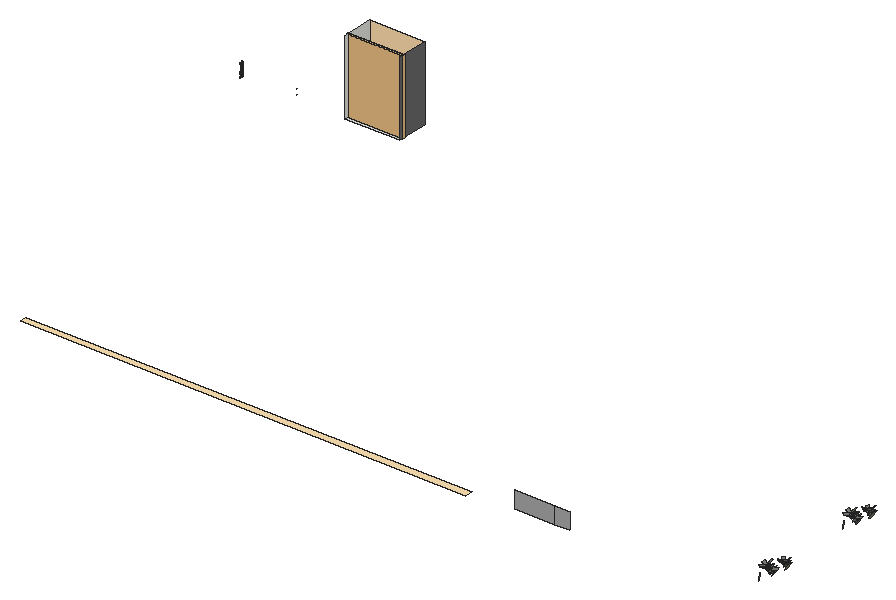
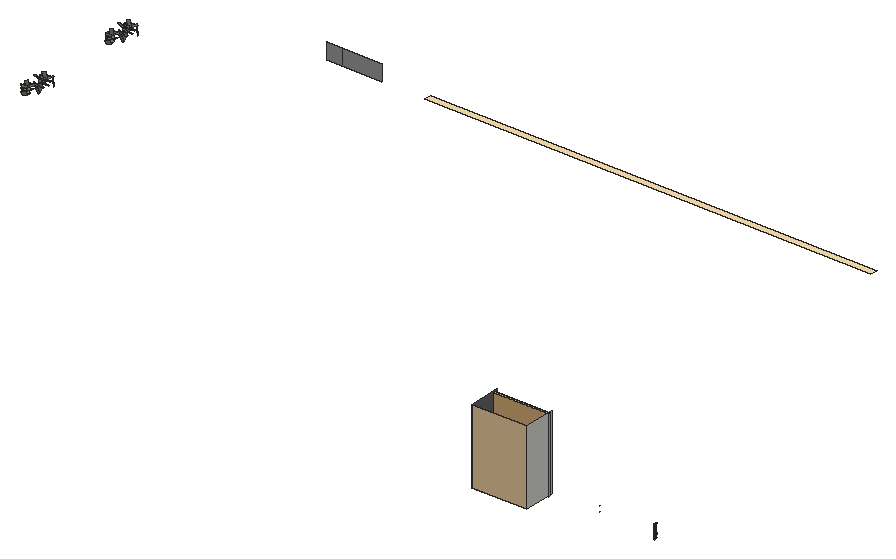
# SketchUp Ruby script. Lengths in inches.
U = 1.inch
M = Sketchup.active_model
def pt(a) = Geom::Point3d.new(a.map { |v| v * U })
def face(e, loops, mat)
  f = e.add_face(loops[0].map { |a| pt(a) })
  loops[1..].each { |l| e.add_face(l.map { |a| pt(a) }).erase! }
  f.material = f.back_material = mat if mat
  f
end
# faces: each face lists its corners as indices into pts; further lists are holes
def faces(e, pts, list, mat = nil) = list.each { |f| face(e, (f[0].is_a?(Array) ? f : [f]).map { |l| l.map { |i| pts[i] } }, mat) }
# xy, xz, yz: faces in a plane at the given z, y or x. An outline is a flat list of corners, or four numbers for a rectangle; further outlines are holes
def ring(l) = l.size == 4 ? [[l[0], l[1]], [l[2], l[1]], [l[2], l[3]], [l[0], l[3]]] : l.each_slice(2).to_a
def flat(e, list, mat, &to3) = list.each { |f| face(e, (f[0].is_a?(Array) ? f : [f]).map { |l| ring(l).map { |u, v| to3.(u, v) } }, mat) }
def xy(e, z, list, mat = nil) = flat(e, list, mat) { |x, y| [x, y, z] }
def xz(e, y, list, mat = nil) = flat(e, list, mat) { |x, z| [x, y, z] }
def yz(e, x, list, mat = nil) = flat(e, list, mat) { |y, z| [x, y, z] }
def lines(e, pts, list) = list.each { |a, b| e.add_line(pt(pts[a]), pt(pts[b])) }
# prism: a flat outline (further loops are holes) pulled along v
def prism(e, loops, v, mat = nil)
  f = face(e, loops, mat); d = Geom::Vector3d.new(v.map { |x| x * U })
  f.pushpull(f.normal.samedirection?(d) ? d.length : -d.length)
end
def box(e, o, s, mat = nil) = prism(e, [[o, [o[0] + s[0], o[1], o[2]], [o[0] + s[0], o[1] + s[1], o[2]], [o[0], o[1] + s[1], o[2]]]], [0, 0, s[2]], mat)
def at(x, y, z, deg = 0) = Geom::Transformation.translation(pt([x, y, z])) * Geom::Transformation.rotation(ORIGIN, Z_AXIS, deg.degrees)
def axes(o, x, y, z) = Geom::Transformation.new([*x, 0, *y, 0, *z, 0, *pt(o).to_a, 1])
def part(name) = M.definitions.add(name)
# library, detail: a bought-in or finely detailed component or shape, given as its bounding box
def library(name, o, s) = part(name).tap { |d| box(d.entities, o, s) }
def detail(e, o, s) = box(e.add_group.entities, o, s)
def put(e, d, t, mat = nil) = e.add_instance(d, t).tap { |i| i.material = mat if mat }
def group(e, t, mat = nil) = e.add_group.tap { |g| g.transformation = t; g.material = mat if mat }.entities
root = M.entities
M.materials.add("Material \#1").color = [140, 140, 140]
M.materials.add("[0032_Moccasin]").color = [255, 228, 181]
M.materials.add("[0033_NavajoWhite]").color = [255, 222, 173]
M.materials.add("[0132_LightGray]").color = [169, 169, 169]
M.materials.add("[0134_DimGray]").color = [105, 105, 105]
M.materials.add("viburnumblaasdfas0df1w06d").color = [98, 102, 84]
M.materials.add("viburnumbladsadfasdfad0w122").color = [125, 129, 119]
c1 = library("Glazed double door",[0,0,0],[5.31,78.43,99.16])
c2 = part("Component\#315")
p = [[0.25,0,0],[2.05,0.01,0.35],[1.81,4.2,1.66],[0,4.19,1.3125]]
faces(c2.entities,p,[[0,1,2,3]],"viburnumbladsadfasdfad0w122")
c3 = part("viburnumblad2")
put(c3.entities,c2,axes([-19.23,-4.49,-32.18],[83.35428,0,0],[0,79.38502,0],[0,0,83.35428]))
c4 = part("Component\#314")
p = [[0.14,0,0],[2.58,0.05,0.25],[2.44,5.11,2.64],[0,5.05,2.39]]
faces(c4.entities,p,[[0,1,2,3]],"viburnumblaasdfas0df1w06d")
c5 = part("viburnumblad1\#2")
put(c5.entities,c4,axes([-37.25,6.23,19.31],[75.98784,0,0],[0,65.50676,0],[0,0,75.98784]))
xy(root,40.75,[[1668.9174,528.0625,1708.7299,550.875]])
xy(root,42.5175,[[1632.1242,529.8706,1632.0426,529.8912,1632.0551,529.9063],[1632.1242,529.8706,1632.0551,529.9063,1632.1285,529.8877],[1632.1242,529.8706,1632.1285,529.8877,1632.211,529.8706],[1632.211,529.8706,1632.1285,529.8877,1632.2067,529.8877],[1632.211,529.8706,1632.2067,529.8877,1632.2926,529.8912],
  [1632.2067,529.8877,1632.2801,529.9063,1632.2926,529.8912],[1632.0426,529.8912,1631.9761,529.93,1631.9953,529.9411],[1632.0426,529.8912,1631.9953,529.9411,1632.0551,529.9063],[1632.2926,529.8912,1632.2801,529.9063,1632.3591,529.93],[1632.2801,529.9063,1632.34,529.9411,1632.3591,529.93],
  [1631.9761,529.93,1631.9327,529.9822,1631.9562,529.9881],[1631.9761,529.93,1631.9562,529.9881,1631.9953,529.9411],[1632.3591,529.93,1632.34,529.9411,1632.4025,529.9822],[1632.34,529.9411,1632.379,529.9881,1632.4025,529.9822],[1631.9327,529.9822,1631.9176,530.0416,1631.9426,530.0416],
  [1631.9327,529.9822,1631.9426,530.0416,1631.9562,529.9881],[1632.4025,529.9822,1632.379,529.9881,1632.4176,530.0416],[1632.379,529.9881,1632.3926,530.0416,1632.4176,530.0416],[1631.9176,530.0416,1631.9327,530.1009,1631.9562,530.095],[1631.9176,530.0416,1631.9562,530.095,1631.9426,530.0416],
  [1632.3926,530.0416,1632.379,530.095,1632.4025,530.1009],[1632.3926,530.0416,1632.4025,530.1009,1632.4176,530.0416],[1631.9562,530.095,1631.9327,530.1009,1631.9953,530.142],[1632.379,530.095,1632.34,530.142,1632.3591,530.1532],[1632.379,530.095,1632.3591,530.1532,1632.4025,530.1009],
  [1631.9327,530.1009,1631.9761,530.1532,1631.9953,530.142],[1631.9953,530.142,1631.9761,530.1532,1632.0551,530.1769],[1632.34,530.142,1632.2801,530.1769,1632.2926,530.1919],[1632.34,530.142,1632.2926,530.1919,1632.3591,530.1532],[1631.9761,530.1532,1632.0426,530.1919,1632.0551,530.1769],
  [1632.0551,530.1769,1632.0426,530.1919,1632.1285,530.1954],[1632.2801,530.1769,1632.2067,530.1954,1632.211,530.2125],[1632.2801,530.1769,1632.211,530.2125,1632.2926,530.1919],[1632.0426,530.1919,1632.1242,530.2125,1632.1285,530.1954],[1632.1285,530.1954,1632.1242,530.2125,1632.2067,530.1954],
  [1632.2067,530.1954,1632.1242,530.2125,1632.211,530.2125]],"Material \#1")
xy(root,42.5353,[[1632.1242,529.8706,1632.1285,529.8877,1632.0426,529.8912],[1632.1242,529.8706,1632.2067,529.8877,1632.1285,529.8877],[1632.1242,529.8706,1632.211,529.8706,1632.2067,529.8877],[1632.211,529.8706,1632.2801,529.9063,1632.2067,529.8877],[1632.211,529.8706,1632.2926,529.8912,1632.2801,529.9063],
  [1632.1285,529.8877,1632.0551,529.9063,1632.0426,529.8912],[1632.0426,529.8912,1632.0551,529.9063,1631.9761,529.93],[1632.2926,529.8912,1632.34,529.9411,1632.2801,529.9063],[1632.2926,529.8912,1632.3591,529.93,1632.34,529.9411],[1632.0551,529.9063,1631.9953,529.9411,1631.9761,529.93],
  [1631.9761,529.93,1631.9953,529.9411,1631.9327,529.9822],[1632.3591,529.93,1632.379,529.9881,1632.34,529.9411],[1632.3591,529.93,1632.4025,529.9822,1632.379,529.9881],[1631.9953,529.9411,1631.9562,529.9881,1631.9327,529.9822],[1631.9327,529.9822,1631.9562,529.9881,1631.9176,530.0416],
  [1632.4025,529.9822,1632.3926,530.0416,1632.379,529.9881],[1632.4025,529.9822,1632.4176,530.0416,1632.3926,530.0416],[1631.9562,529.9881,1631.9426,530.0416,1631.9176,530.0416],[1631.9176,530.0416,1631.9426,530.0416,1631.9327,530.1009],[1631.9426,530.0416,1631.9562,530.095,1631.9327,530.1009],
  [1632.3926,530.0416,1632.4176,530.0416,1632.379,530.095],[1632.4176,530.0416,1632.4025,530.1009,1632.379,530.095],[1631.9562,530.095,1631.9761,530.1532,1631.9327,530.1009],[1631.9562,530.095,1631.9953,530.142,1631.9761,530.1532],[1632.379,530.095,1632.4025,530.1009,1632.34,530.142],
  [1632.4025,530.1009,1632.3591,530.1532,1632.34,530.142],[1631.9953,530.142,1632.0426,530.1919,1631.9761,530.1532],[1631.9953,530.142,1632.0551,530.1769,1632.0426,530.1919],[1632.34,530.142,1632.3591,530.1532,1632.2801,530.1769],[1632.3591,530.1532,1632.2926,530.1919,1632.2801,530.1769],
  [1632.0551,530.1769,1632.1242,530.2125,1632.0426,530.1919],[1632.0551,530.1769,1632.1285,530.1954,1632.1242,530.2125],[1632.2801,530.1769,1632.2926,530.1919,1632.2067,530.1954],[1632.2926,530.1919,1632.211,530.2125,1632.2067,530.1954],[1632.1285,530.1954,1632.211,530.2125,1632.1242,530.2125],
  [1632.1285,530.1954,1632.2067,530.1954,1632.211,530.2125]],"Material \#1")
xy(root,46.5278,[[1632.1242,529.8706,1632.0426,529.8912,1632.1286,529.8877],[1632.1242,529.8706,1632.1286,529.8877,1632.2067,529.8877],[1632.1242,529.8706,1632.2067,529.8877,1632.211,529.8706],[1632.211,529.8706,1632.2067,529.8877,1632.2801,529.9063],[1632.211,529.8706,1632.2801,529.9063,1632.2926,529.8912],
  [1632.1286,529.8877,1632.0426,529.8912,1632.0551,529.9063],[1632.0426,529.8912,1631.9761,529.93,1632.0551,529.9063],[1632.2926,529.8912,1632.2801,529.9063,1632.34,529.9411],[1632.2926,529.8912,1632.34,529.9411,1632.3591,529.93],[1632.0551,529.9063,1631.9761,529.93,1631.9953,529.9411],
  [1631.9761,529.93,1631.9327,529.9822,1631.9953,529.9411],[1632.3591,529.93,1632.34,529.9411,1632.379,529.9881],[1632.3591,529.93,1632.379,529.9881,1632.4025,529.9822],[1631.9953,529.9411,1631.9327,529.9822,1631.9562,529.9881],[1631.9327,529.9822,1631.9176,530.0416,1631.9562,529.9881],
  [1632.4025,529.9822,1632.379,529.9881,1632.3926,530.0416],[1632.4025,529.9822,1632.3926,530.0416,1632.4176,530.0416],[1631.9562,529.9881,1631.9176,530.0416,1631.9426,530.0416],[1631.9176,530.0416,1631.9327,530.1009,1631.9426,530.0416],[1631.9426,530.0416,1631.9327,530.1009,1631.9562,530.095],
  [1632.3926,530.0416,1632.379,530.095,1632.4176,530.0416],[1632.4176,530.0416,1632.379,530.095,1632.4025,530.1009],[1631.9562,530.095,1631.9327,530.1009,1631.9761,530.1532],[1631.9562,530.095,1631.9761,530.1532,1631.9953,530.142],[1632.379,530.095,1632.34,530.142,1632.4025,530.1009],
  [1632.4025,530.1009,1632.34,530.142,1632.3591,530.1532],[1631.9953,530.142,1631.9761,530.1532,1632.0426,530.1919],[1631.9953,530.142,1632.0426,530.1919,1632.0551,530.1769],[1632.34,530.142,1632.2801,530.1769,1632.3591,530.1532],[1632.3591,530.1532,1632.2801,530.1769,1632.2926,530.1919],
  [1632.0551,530.1769,1632.0426,530.1919,1632.1242,530.2125],[1632.0551,530.1769,1632.1242,530.2125,1632.1286,530.1954],[1632.2801,530.1769,1632.2067,530.1954,1632.2926,530.1919],[1632.2926,530.1919,1632.2067,530.1954,1632.211,530.2125],[1632.1286,530.1954,1632.1242,530.2125,1632.211,530.2125],
  [1632.1286,530.1954,1632.211,530.2125,1632.2067,530.1954]],"Material \#1")
xy(root,46.5456,[[1632.1242,529.8706,1632.0551,529.9063,1632.0426,529.8912],[1632.1242,529.8706,1632.1286,529.8877,1632.0551,529.9063],[1632.1242,529.8706,1632.211,529.8706,1632.1286,529.8877],[1632.211,529.8706,1632.2067,529.8877,1632.1286,529.8877],[1632.211,529.8706,1632.2926,529.8912,1632.2067,529.8877],
  [1632.2067,529.8877,1632.2926,529.8912,1632.2801,529.9063],[1632.0426,529.8912,1631.9953,529.9411,1631.9761,529.93],[1632.0426,529.8912,1632.0551,529.9063,1631.9953,529.9411],[1632.2926,529.8912,1632.3591,529.93,1632.2801,529.9063],[1632.2801,529.9063,1632.3591,529.93,1632.34,529.9411],
  [1631.9761,529.93,1631.9562,529.9881,1631.9327,529.9822],[1631.9761,529.93,1631.9953,529.9411,1631.9562,529.9881],[1632.3591,529.93,1632.4025,529.9822,1632.34,529.9411],[1632.34,529.9411,1632.4025,529.9822,1632.379,529.9881],[1631.9327,529.9822,1631.9426,530.0416,1631.9176,530.0416],
  [1631.9327,529.9822,1631.9562,529.9881,1631.9426,530.0416],[1632.4025,529.9822,1632.4176,530.0416,1632.379,529.9881],[1632.379,529.9881,1632.4176,530.0416,1632.3926,530.0416],[1631.9176,530.0416,1631.9426,530.0416,1631.9562,530.095],[1631.9176,530.0416,1631.9562,530.095,1631.9327,530.1009],
  [1632.3926,530.0416,1632.4025,530.1009,1632.379,530.095],[1632.3926,530.0416,1632.4176,530.0416,1632.4025,530.1009],[1631.9562,530.095,1631.9953,530.142,1631.9327,530.1009],[1632.379,530.095,1632.3591,530.1532,1632.34,530.142],[1632.379,530.095,1632.4025,530.1009,1632.3591,530.1532],
  [1631.9327,530.1009,1631.9953,530.142,1631.9761,530.1532],[1631.9953,530.142,1632.0551,530.1769,1631.9761,530.1532],[1632.34,530.142,1632.2926,530.1919,1632.2801,530.1769],[1632.34,530.142,1632.3591,530.1532,1632.2926,530.1919],[1631.9761,530.1532,1632.0551,530.1769,1632.0426,530.1919],
  [1632.0551,530.1769,1632.1286,530.1954,1632.0426,530.1919],[1632.2801,530.1769,1632.211,530.2125,1632.2067,530.1954],[1632.2801,530.1769,1632.2926,530.1919,1632.211,530.2125],[1632.0426,530.1919,1632.1286,530.1954,1632.1242,530.2125],[1632.1286,530.1954,1632.2067,530.1954,1632.1242,530.2125],
  [1632.2067,530.1954,1632.211,530.2125,1632.1242,530.2125]],"Material \#1")
xy(root,47.6814,[[1678.9389,218.9375,2004.7084,223.9375]],"[0032_Moccasin]")
xz(root,223.9375,[[2036.3125,48,2065.6875,60]],"[0132_LightGray]")
xz(root,529.3124,[[1591.1102,42.1281,1591.052,42.4891,1591.1077,42.5206],[1591.1102,42.1281,1591.1077,42.5206,1591.1102,42.4516],[1591.1102,42.4516,1591.1077,42.5206,1591.1121,42.4659],[1591.1102,42.4516,1591.1121,42.4659,1591.1107,42.4591],[1591.1121,42.4659,1591.1077,42.5206,1591.1542,42.562],
  [1591.1121,42.4659,1591.1179,42.478,1591.1145,42.4721],[1591.1121,42.4659,1591.1542,42.562,1591.1179,42.478],[1591.1179,42.478,1591.1542,42.562,1591.1896,42.6116],[1591.1179,42.478,1591.1896,42.6116,1591.2571,42.6891],[1591.1179,42.478,1591.2571,42.6891,1591.1221,42.4835],
  [1591.1221,42.4835,1591.2571,42.6891,1591.1273,42.4887],[1591.1273,42.4887,1591.1913,42.549,1591.1333,42.4937],[1591.1273,42.4887,1591.2571,42.6891,1591.1913,42.549],[1591.1333,42.4937,1591.1913,42.549,1591.164,42.52],[1591.1913,42.549,1591.2339,42.6147,1591.2148,42.5807],
  [1591.1913,42.549,1591.2571,42.6891,1591.2339,42.6147],[1591.1896,42.6116,1591.2122,42.6678,1591.2571,42.6891],[1591.2339,42.6147,1591.2571,42.6891,1591.2482,42.6509],[1591.2122,42.6678,1591.2202,42.729,1591.2571,42.6891],[1591.2571,42.6891,1591.1854,42.9182,1591.2512,42.7983],
  [1591.2571,42.6891,1591.1896,42.8463,1591.1854,42.9182],[1591.2571,42.6891,1591.2122,42.7902,1591.1896,42.8463],[1591.2571,42.6891,1591.2202,42.729,1591.2122,42.7902],[1591.2571,42.6891,1591.2512,42.7983,1591.2602,42.7289],[1591.2512,42.7983,1591.1854,42.9182,1591.2256,42.862],
  [1591.1896,42.8463,1591.1542,42.8959,1591.1854,42.9182],[1591.1542,42.8959,1591.1077,42.9373,1591.1854,42.9182],[1591.1854,42.9182,1590.9202,43.0316,1591.0696,43.0008],[1591.1854,42.9182,1591.052,42.9688,1590.9202,43.0316],[1591.1854,42.9182,1591.1077,42.9373,1591.052,42.9688],
  [1591.1854,42.9182,1591.0696,43.0008,1591.1327,42.9651]],"Material \#1")
xz(root,529.3472,[[1591.1073,39.5491,1591.0976,39.5594,1591.1308,39.5889],[1591.1073,39.5491,1591.1308,39.5889,1591.1423,39.5802],[1591.5889,39.557,1591.5774,39.5657,1591.6622,39.6725],[1591.5889,39.557,1591.6622,39.6725,1591.6752,39.6657],[1591.1423,39.5802,1591.1308,39.5889,1591.1579,39.6231],
  [1591.1423,39.5802,1591.1579,39.6231,1591.1709,39.6163],[1591.1709,39.6163,1591.1579,39.6231,1591.1784,39.6614],[1591.1709,39.6163,1591.1784,39.6614,1591.1925,39.6567],[1591.1925,39.6567,1591.1784,39.6614,1591.1912,39.703],[1591.1925,39.6567,1591.1912,39.703,1591.2061,39.7006],
  [1591.6752,39.6657,1591.6622,39.6725,1591.7258,39.7916],[1591.6752,39.6657,1591.7258,39.7916,1591.7399,39.7869],[1591.2061,39.7006,1591.1912,39.703,1591.1957,39.7468],[1591.2061,39.7006,1591.1957,39.7468,1591.2107,39.7468],[1591.1957,39.7468,1591.1912,39.7907,1591.2107,39.7468],
  [1591.2107,39.7468,1591.1912,39.7907,1591.2061,39.7931],[1591.7399,39.7869,1591.7258,39.7916,1591.7657,39.9208],[1591.7399,39.7869,1591.7657,39.9208,1591.7805,39.9184],[1591.1912,39.7907,1591.1784,39.8323,1591.2061,39.7931],[1591.2061,39.7931,1591.1784,39.8323,1591.1925,39.837],
  [1591.1784,39.8323,1591.1579,39.8706,1591.1925,39.837],[1591.1925,39.837,1591.1579,39.8706,1591.1709,39.8774],[1591.1579,39.8706,1591.1308,39.9048,1591.1709,39.8774],[1591.1709,39.8774,1591.1308,39.9048,1591.1423,39.9135],[1591.1308,39.9048,1591.0976,39.9343,1591.1423,39.9135],
  [1591.1423,39.9135,1591.0976,39.9343,1591.1073,39.9446],[1591.7805,39.9184,1591.7657,39.9208,1591.7801,40.064],[1591.7805,39.9184,1591.7801,40.064,1591.7951,40.0634],[1591.0976,39.9343,1591.0592,39.9585,1591.1073,39.9446],[1591.1073,39.9446,1591.0592,39.9585,1591.0668,39.9701],
  [1591.7951,40.0634,1591.7801,40.064,1591.7801,47.0385],[1591.7951,40.0634,1591.7801,47.0385,1591.7801,48.9547],[1591.7951,40.0634,1591.7801,48.9547,1591.7951,48.9553],[1591.7801,48.9547,1591.7657,49.0979,1591.7951,48.9553],[1591.7951,48.9553,1591.7657,49.0979,1591.7805,49.1003],
  [1591.0668,49.0486,1591.0592,49.0602,1591.0976,49.0844],[1591.0668,49.0486,1591.0976,49.0844,1591.1073,49.0741],[1591.1073,49.0741,1591.0976,49.0844,1591.1308,49.1139],[1591.1073,49.0741,1591.1308,49.1139,1591.1423,49.1052],[1591.7657,49.0979,1591.7258,49.2271,1591.7805,49.1003],
  [1591.7805,49.1003,1591.7258,49.2271,1591.7399,49.2318],[1591.1423,49.1052,1591.1308,49.1139,1591.1579,49.1481],[1591.1423,49.1052,1591.1579,49.1481,1591.1709,49.1413],[1591.1709,49.1413,1591.1579,49.1481,1591.1784,49.1863],[1591.1709,49.1413,1591.1784,49.1863,1591.1925,49.1817],
  [1591.1925,49.1817,1591.1784,49.1863,1591.1912,49.228],[1591.1925,49.1817,1591.1912,49.228,1591.2061,49.2256],[1591.2061,49.2256,1591.1912,49.228,1591.1957,49.2718],[1591.2061,49.2256,1591.1957,49.2718,1591.2107,49.2718],[1591.7258,49.2271,1591.6622,49.3462,1591.7399,49.2318],
  [1591.7399,49.2318,1591.6622,49.3462,1591.6752,49.3529],[1591.1957,49.2718,1591.1912,49.3157,1591.2107,49.2718],[1591.2107,49.2718,1591.1912,49.3157,1591.2061,49.3181],[1591.1912,49.3157,1591.1784,49.3573,1591.2061,49.3181],[1591.2061,49.3181,1591.1784,49.3573,1591.1925,49.362],
  [1591.6622,49.3462,1591.5774,49.453,1591.6752,49.3529],[1591.6752,49.3529,1591.5774,49.453,1591.5889,49.4616],[1591.1784,49.3573,1591.1579,49.3956,1591.1925,49.362],[1591.1925,49.362,1591.1579,49.3956,1591.1709,49.4024],[1591.1579,49.3956,1591.1308,49.4298,1591.1709,49.4024],
  [1591.1709,49.4024,1591.1308,49.4298,1591.1423,49.4385],[1591.1308,49.4298,1591.0976,49.4593,1591.1423,49.4385],[1591.1423,49.4385,1591.0976,49.4593,1591.1073,49.4696],[1591.5774,49.453,1591.4737,49.5453,1591.5889,49.4616],[1591.0976,49.4593,1591.0592,49.4835,1591.1073,49.4696],
  [1591.5889,49.4616,1591.4737,49.5453,1591.4834,49.5556],[1591.1073,49.4696,1591.0592,49.4835,1591.0668,49.4951],[1591.4737,49.5453,1591.3537,49.6209,1591.4834,49.5556],[1591.4834,49.5556,1591.3537,49.6209,1591.3613,49.6324],[1591.3537,49.6209,1591.2199,49.6774,1591.3613,49.6324],
  [1591.3613,49.6324,1591.2199,49.6774,1591.2252,49.69],[1591.2199,49.6774,1591.0748,49.713,1591.2252,49.69],[1591.2252,49.69,1591.0748,49.713,1591.0775,49.7262]],"Material \#1")
xz(root,529.6596,[[1591.0037,41.9762,1591.0684,42.0223,1591.1051,42.0894],[1591.0684,42.0223,1591.0908,42.0538,1591.1051,42.0894],[1591.1102,42.1281,1591.1102,42.4516,1590.9889,42.469],[1591.1102,42.4516,1591.1121,42.4659,1590.9889,42.469],[1591.1102,42.4516,1591.1107,42.4591,1591.1121,42.4659],
  [1591.1121,42.4659,1591.1179,42.478,1590.9889,42.469],[1591.1121,42.4659,1591.1145,42.4721,1591.1179,42.478],[1590.9889,42.469,1591.1179,42.478,1591.052,42.4891],[1591.1179,42.478,1591.1077,42.5206,1591.052,42.4891],[1591.1179,42.478,1591.1542,42.562,1591.1077,42.5206],
  [1591.1179,42.478,1591.1221,42.4835,1591.2571,42.6891],[1591.1179,42.478,1591.2571,42.6891,1591.1542,42.562],[1591.1221,42.4835,1591.1273,42.4887,1591.2571,42.6891],[1591.1273,42.4887,1591.1333,42.4937,1591.1913,42.549],[1591.1273,42.4887,1591.1913,42.549,1591.2571,42.6891],
  [1591.1333,42.4937,1591.164,42.52,1591.1913,42.549],[1591.1913,42.549,1591.2148,42.5807,1591.2339,42.6147],[1591.1913,42.549,1591.2339,42.6147,1591.2571,42.6891],[1591.1542,42.562,1591.2571,42.6891,1591.1896,42.6116],[1591.1896,42.6116,1591.2571,42.6891,1591.2122,42.6678],
  [1591.2339,42.6147,1591.2482,42.6509,1591.2571,42.6891],[1591.2122,42.6678,1591.2571,42.6891,1591.2202,42.729],[1591.2571,42.6891,1591.1854,42.9182,1591.2122,42.7902],[1591.2571,42.6891,1591.2512,42.7983,1591.1854,42.9182],[1591.2571,42.6891,1591.2122,42.7902,1591.2202,42.729],
  [1591.2571,42.6891,1591.2602,42.7289,1591.2512,42.7983],[1591.2122,42.7902,1591.1854,42.9182,1591.1896,42.8463],[1591.2512,42.7983,1591.2256,42.862,1591.1854,42.9182],[1591.1896,42.8463,1591.1854,42.9182,1591.1542,42.8959],[1591.1542,42.8959,1591.1854,42.9182,1591.1077,42.9373],
  [1591.1854,42.9182,1591.0696,43.0008,1590.9202,43.0316],[1591.1854,42.9182,1591.052,42.9688,1591.1077,42.9373],[1591.1854,42.9182,1591.1327,42.9651,1591.0696,43.0008]],"Material \#1")
xz(root,531.0484,[[1591.0037,41.9762,1591.1051,42.0894,1591.0684,42.0223],[1591.0684,42.0223,1591.1051,42.0894,1591.0908,42.0538],[1591.1102,42.1281,1590.9889,42.469,1591.1102,42.4517],[1591.1102,42.4517,1590.9889,42.469,1591.1121,42.4659],[1591.1102,42.4517,1591.1121,42.4659,1591.1107,42.4591],
  [1591.1121,42.4659,1590.9889,42.469,1591.1179,42.478],[1591.1121,42.4659,1591.1179,42.478,1591.1145,42.4721],[1590.9889,42.469,1591.052,42.4891,1591.1179,42.478],[1591.1179,42.478,1591.052,42.4891,1591.1077,42.5206],[1591.1179,42.478,1591.1077,42.5206,1591.1542,42.562],
  [1591.1179,42.478,1591.1542,42.562,1591.2571,42.6891],[1591.1179,42.478,1591.2571,42.6891,1591.1221,42.4835],[1591.1221,42.4835,1591.2571,42.6891,1591.1273,42.4887],[1591.1273,42.4887,1591.1913,42.549,1591.1333,42.4937],[1591.1273,42.4887,1591.2571,42.6891,1591.1913,42.549],
  [1591.1333,42.4937,1591.1913,42.549,1591.164,42.52],[1591.1913,42.549,1591.2339,42.6147,1591.2148,42.5807],[1591.1913,42.549,1591.2571,42.6891,1591.2339,42.6147],[1591.1542,42.562,1591.1896,42.6116,1591.2571,42.6891],[1591.1896,42.6116,1591.2122,42.6678,1591.2571,42.6891],
  [1591.2339,42.6147,1591.2571,42.6891,1591.2482,42.6509],[1591.2122,42.6678,1591.2202,42.729,1591.2571,42.6891],[1591.2571,42.6891,1591.1854,42.9182,1591.2512,42.7983],[1591.2571,42.6891,1591.2122,42.7902,1591.1854,42.9182],[1591.2571,42.6891,1591.2202,42.729,1591.2122,42.7902],
  [1591.2571,42.6891,1591.2512,42.7983,1591.2602,42.7289],[1591.2122,42.7902,1591.1896,42.8463,1591.1854,42.9182],[1591.2512,42.7983,1591.1854,42.9182,1591.2256,42.862],[1591.1896,42.8463,1591.1542,42.8959,1591.1854,42.9182],[1591.1542,42.8959,1591.1077,42.9373,1591.1854,42.9182],
  [1591.1854,42.9182,1590.9202,43.0316,1591.0696,43.0008],[1591.1854,42.9182,1591.1077,42.9373,1591.052,42.9688],[1591.1854,42.9182,1591.0696,43.0008,1591.1327,42.9651]],"Material \#1")
xz(root,531.3609,[[1591.0668,39.5236,1591.0976,39.5594,1591.0592,39.5352],[1591.0668,39.5236,1591.1073,39.5491,1591.0976,39.5594],[1591.1073,39.5491,1591.1308,39.5889,1591.0976,39.5594],[1591.1073,39.5491,1591.1423,39.5802,1591.1308,39.5889],[1591.5889,39.557,1591.6622,39.6725,1591.5774,39.5657],
  [1591.5889,39.557,1591.6752,39.6657,1591.6622,39.6725],[1591.1423,39.5802,1591.1579,39.6231,1591.1308,39.5889],[1591.1423,39.5802,1591.1709,39.6163,1591.1579,39.6231],[1591.1709,39.6163,1591.1784,39.6614,1591.1579,39.6231],[1591.1709,39.6163,1591.1925,39.6567,1591.1784,39.6614],
  [1591.1925,39.6567,1591.1912,39.703,1591.1784,39.6614],[1591.1925,39.6567,1591.2061,39.7006,1591.1912,39.703],[1591.6752,39.6657,1591.7258,39.7916,1591.6622,39.6725],[1591.6752,39.6657,1591.7399,39.7869,1591.7258,39.7916],[1591.2061,39.7006,1591.1957,39.7468,1591.1912,39.703],
  [1591.2061,39.7006,1591.2107,39.7468,1591.1957,39.7468],[1591.1957,39.7468,1591.2107,39.7468,1591.1912,39.7907],[1591.2107,39.7468,1591.2061,39.7931,1591.1912,39.7907],[1591.7399,39.7869,1591.7657,39.9208,1591.7258,39.7916],[1591.7399,39.7869,1591.7805,39.9184,1591.7657,39.9208],
  [1591.1912,39.7907,1591.2061,39.7931,1591.1784,39.8323],[1591.2061,39.7931,1591.1925,39.837,1591.1784,39.8323],[1591.1784,39.8323,1591.1925,39.837,1591.1579,39.8706],[1591.1925,39.837,1591.1709,39.8774,1591.1579,39.8706],[1591.1579,39.8706,1591.1709,39.8774,1591.1308,39.9048],
  [1591.1709,39.8774,1591.1423,39.9135,1591.1308,39.9048],[1591.1308,39.9048,1591.1423,39.9135,1591.0976,39.9343],[1591.1423,39.9135,1591.1073,39.9446,1591.0976,39.9343],[1591.7805,39.9184,1591.7801,40.064,1591.7657,39.9208],[1591.7805,39.9184,1591.7951,40.0634,1591.7801,40.064],
  [1591.0976,39.9343,1591.1073,39.9446,1591.0592,39.9585],[1591.1073,39.9446,1591.0668,39.9701,1591.0592,39.9585],[1591.7951,40.0634,1591.7801,47.0385,1591.7801,40.064],[1591.7951,40.0634,1591.7801,48.9547,1591.7801,47.0385],[1591.7951,40.0634,1591.7951,48.9553,1591.7801,48.9547],
  [1591.7801,48.9547,1591.7951,48.9553,1591.7657,49.0979],[1591.7951,48.9553,1591.7805,49.1003,1591.7657,49.0979],[1591.0668,49.0486,1591.0976,49.0844,1591.0592,49.0602],[1591.0668,49.0486,1591.1073,49.0741,1591.0976,49.0844],[1591.1073,49.0741,1591.1308,49.1138,1591.0976,49.0844],
  [1591.1073,49.0741,1591.1423,49.1052,1591.1308,49.1138],[1591.7657,49.0979,1591.7805,49.1003,1591.7258,49.2271],[1591.7805,49.1003,1591.7399,49.2318,1591.7258,49.2271],[1591.1423,49.1052,1591.1579,49.1481,1591.1308,49.1138],[1591.1423,49.1052,1591.1709,49.1413,1591.1579,49.1481],
  [1591.1709,49.1413,1591.1784,49.1863,1591.1579,49.1481],[1591.1709,49.1413,1591.1925,49.1817,1591.1784,49.1863],[1591.1925,49.1817,1591.1912,49.228,1591.1784,49.1863],[1591.1925,49.1817,1591.2061,49.2256,1591.1912,49.228],[1591.2061,49.2256,1591.1957,49.2718,1591.1912,49.228],
  [1591.2061,49.2256,1591.2107,49.2718,1591.1957,49.2718],[1591.7258,49.2271,1591.7399,49.2318,1591.6622,49.3462],[1591.7399,49.2318,1591.6752,49.3529,1591.6622,49.3462],[1591.1957,49.2718,1591.2107,49.2718,1591.1912,49.3157],[1591.2107,49.2718,1591.2061,49.3181,1591.1912,49.3157],
  [1591.1912,49.3157,1591.2061,49.3181,1591.1784,49.3573],[1591.2061,49.3181,1591.1925,49.362,1591.1784,49.3573],[1591.6622,49.3462,1591.6752,49.3529,1591.5774,49.453],[1591.6752,49.3529,1591.5889,49.4616,1591.5774,49.453],[1591.1784,49.3573,1591.1925,49.362,1591.1579,49.3956],
  [1591.1925,49.362,1591.1709,49.4024,1591.1579,49.3956],[1591.1579,49.3956,1591.1709,49.4024,1591.1308,49.4298],[1591.1709,49.4024,1591.1423,49.4385,1591.1308,49.4298],[1591.1308,49.4298,1591.1423,49.4385,1591.0976,49.4593],[1591.1423,49.4385,1591.1073,49.4696,1591.0976,49.4593],
  [1591.5774,49.453,1591.5889,49.4616,1591.4737,49.5453],[1591.0976,49.4593,1591.1073,49.4696,1591.0592,49.4835],[1591.5889,49.4616,1591.4834,49.5556,1591.4737,49.5453],[1591.1073,49.4696,1591.0668,49.4951,1591.0592,49.4835],[1591.4737,49.5453,1591.4834,49.5556,1591.3537,49.6209],
  [1591.4834,49.5556,1591.3613,49.6324,1591.3537,49.6209],[1591.3537,49.6209,1591.3613,49.6324,1591.2199,49.6774],[1591.3613,49.6324,1591.2252,49.69,1591.2199,49.6774],[1591.2199,49.6774,1591.2252,49.69,1591.0748,49.713],[1591.2252,49.69,1591.0775,49.7262,1591.0748,49.713]],"Material \#1")
xz(root,531.3956,[[1591.0684,42.0223,1591.0908,42.0538,1591.1051,42.0894],[1591.0684,42.0223,1591.1051,42.0894,1591.1102,42.1281],[1591.1102,42.1281,1591.1077,42.5206,1591.052,42.4891],[1591.1102,42.1281,1591.1102,42.4517,1591.1077,42.5206],[1591.1102,42.4517,1591.1121,42.4659,1591.1077,42.5206],
  [1591.1102,42.4517,1591.1107,42.4591,1591.1121,42.4659],[1591.1121,42.4659,1591.1542,42.562,1591.1077,42.5206],[1591.1121,42.4659,1591.1145,42.4721,1591.1179,42.478],[1591.1121,42.4659,1591.1179,42.478,1591.1542,42.562],[1591.1179,42.478,1591.1221,42.4835,1591.2571,42.6891],
  [1591.1179,42.478,1591.1896,42.6116,1591.1542,42.562],[1591.1179,42.478,1591.2571,42.6891,1591.1896,42.6116],[1591.1221,42.4835,1591.1273,42.4887,1591.2571,42.6891],[1591.1273,42.4887,1591.1333,42.4937,1591.1913,42.549],[1591.1273,42.4887,1591.1913,42.549,1591.2571,42.6891],
  [1591.1333,42.4937,1591.164,42.52,1591.1913,42.549],[1591.1913,42.549,1591.2148,42.5807,1591.2339,42.6147],[1591.1913,42.549,1591.2339,42.6147,1591.2571,42.6891],[1591.1896,42.6116,1591.2571,42.6891,1591.2122,42.6678],[1591.2339,42.6147,1591.2482,42.6509,1591.2571,42.6891],
  [1591.2122,42.6678,1591.2571,42.6891,1591.2202,42.729],[1591.2571,42.6891,1591.1854,42.9182,1591.1896,42.8463],[1591.2571,42.6891,1591.2512,42.7983,1591.1854,42.9182],[1591.2571,42.6891,1591.1896,42.8463,1591.2122,42.7902],[1591.2571,42.6891,1591.2122,42.7902,1591.2202,42.729],
  [1591.2571,42.6891,1591.2602,42.7289,1591.2512,42.7983],[1591.2512,42.7983,1591.2256,42.862,1591.1854,42.9182],[1591.1896,42.8463,1591.1854,42.9182,1591.1542,42.8959],[1591.1542,42.8959,1591.1854,42.9182,1591.1077,42.9373],[1591.1854,42.9182,1590.9202,43.0316,1591.052,42.9688],
  [1591.1854,42.9182,1591.0696,43.0008,1590.9202,43.0316],[1591.1854,42.9182,1591.052,42.9688,1591.1077,42.9373],[1591.1854,42.9182,1591.1327,42.9651,1591.0696,43.0008]],"Material \#1")
xz(root,550.875,[[1668.9174,40.75,1708.7299,95.25]],"[0033_NavajoWhite]")
yz(root,1668.9174,[[528.0625,40.75,550.875,95.25]])
yz(root,1708.7299,[[528.0625,40.75,550.875,95.25]],"[0134_DimGray]")
p = [[2065.6875,223.9375,60],[2065.6875,223.9375,48],[2076.625,224.2109,48],[2076.625,224.2109,60]]
faces(root,p,[[0,1,2,3]],"[0132_LightGray]")
put(root,c1,axes([1709.4375,530.58,40.75],[0,0.25,0],[-0.525,0,0],[0,0,0.54963]))
put(root,c3,axes([2188.35,339.5,47.25],[0.00639,0.01034,0.00318],[-0.01046,0.00683,-0.00122],[-0.00247,-0.00201,0.01151]))
put(root,c3,axes([2188.35,262.61,47.25],[0.00639,0.01034,0.00318],[-0.01046,0.00683,-0.00122],[-0.00247,-0.00201,0.01151]))
put(root,c3,axes([2189.74,339.4,46.09],[-0.00261,0.01228,0.0004],[-0.01201,-0.00247,-0.00269],[-0.00228,-0.00087,0.01169]))
put(root,c3,axes([2189.74,262.52,46.09],[-0.00261,0.01228,0.0004],[-0.01201,-0.00247,-0.00269],[-0.00228,-0.00087,0.01169]))
put(root,c3,axes([2189.86,339.52,47.75],[-0.01008,0.00703,-0.00261],[-0.00679,-0.01041,-0.00178],[-0.00292,0.0001,0.01158]))
put(root,c3,axes([2189.86,262.64,47.75],[-0.01008,0.00703,-0.00261],[-0.00679,-0.01041,-0.00178],[-0.00292,0.0001,0.01158]))
put(root,c3,axes([2189.65,339.85,44.55],[0.00613,0.00993,0.00305],[-0.0113,0.00738,-0.00131],[-0.00247,-0.00201,0.01151]))
put(root,c3,axes([2189.65,262.96,44.55],[0.00613,0.00993,0.00305],[-0.0113,0.00738,-0.00131],[-0.00247,-0.00201,0.01151]))
put(root,c3,axes([2187.35,334.57,40.19],[0.00935,-0.00836,0.00053],[0.0036,0.00454,0.01078],[-0.00748,-0.0082,0.00525]))
put(root,c3,axes([2187.35,257.6875,40.19],[0.00935,-0.00836,0.00053],[0.0036,0.00454,0.01078],[-0.00748,-0.0082,0.00525]))
put(root,c3,axes([2188.67,340.3,45.81],[0.01164,0.00234,0.00409],[-0.0032,0.01265,0.00186],[-0.00338,-0.00265,0.01114]))
put(root,c3,axes([2188.67,263.41,45.81],[0.01164,0.00234,0.00409],[-0.0032,0.01265,0.00186],[-0.00338,-0.00265,0.01114]))
put(root,c3,axes([2188.28,341.07,47.39],[0.01008,-0.00703,0.00261],[0.00588,0.01012,0.00453],[-0.00448,-0.00242,0.01081]))
put(root,c3,axes([2188.28,264.19,47.39],[0.01008,-0.00703,0.00261],[0.00588,0.01012,0.00453],[-0.00448,-0.00242,0.01081]))
put(root,c5,axes([2190.03,341.22,41.67],[0.01199,-0.00124,0.00662],[-0.00048,0.01553,0.00369],[-0.00665,-0.00299,0.01093]))
put(root,c5,axes([2190.03,264.34,41.67],[0.01199,-0.00124,0.00662],[-0.00048,0.01553,0.00369],[-0.00665,-0.00299,0.01093]))
put(root,c3,axes([2189.16,346.43,40.44],[0.00637,-0.00937,0.00151],[0.00514,0.00494,0.00894],[-0.00798,-0.0043,0.00697]))
put(root,c3,axes([2189.16,269.55,40.44],[0.00637,-0.00937,0.00151],[0.00514,0.00494,0.00894],[-0.00798,-0.0043,0.00697]))
put(root,c3,axes([2190.74,340.58,46.54],[-0.01164,-0.00234,-0.00409],[0.00216,-0.01246,0.00098],[-0.00402,0.00034,0.01124]))
put(root,c3,axes([2190.74,263.7,46.54],[-0.01164,-0.00234,-0.00409],[0.00216,-0.01246,0.00098],[-0.00402,0.00034,0.01124]))
put(root,c3,axes([2190.26,345.85,41.18],[-0.00608,-0.00542,-0.00802],[0.00543,-0.00975,0.00248],[-0.00802,-0.0025,0.00776]))
put(root,c3,axes([2190.26,268.97,41.18],[-0.00608,-0.00542,-0.00802],[0.00543,-0.00975,0.00248],[-0.00802,-0.0025,0.00776]))
put(root,c3,axes([2189.79,341.1,47.89],[-0.00639,-0.01034,-0.00318],[0.00955,-0.00712,0.00396],[-0.00493,-0.0003,0.01087]))
put(root,c3,axes([2189.79,264.22,47.89],[-0.00639,-0.01034,-0.00318],[0.00955,-0.00712,0.00396],[-0.00493,-0.0003,0.01087]))
put(root,c3,axes([2189.43,341.42,44.68],[0.01052,-0.00734,0.00272],[0.0053,0.00911,0.00408],[-0.00448,-0.00242,0.01081]))
put(root,c3,axes([2189.43,264.54,44.68],[0.01052,-0.00734,0.00272],[0.0053,0.00911,0.00408],[-0.00448,-0.00242,0.01081]))
put(root,c3,axes([2189.33,341.58,46.14],[0.00261,-0.01228,-0.0004],[0.01019,0.002,0.00499],[-0.00512,-0.00144,0.01069]))
put(root,c3,axes([2189.33,264.69,46.14],[0.00261,-0.01228,-0.0004],[0.01019,0.002,0.00499],[-0.00512,-0.00144,0.01069]))
put(root,c3,axes([2191.78,351.67,46],[0.00825,0.0079,0.00055],[-0.00775,0.00821,-0.00179],[-0.00163,0.00092,0.01128]))
put(root,c3,axes([2191.78,274.79,46],[0.00825,0.0079,0.00055],[-0.00775,0.00821,-0.00179],[-0.00163,0.00092,0.01128]))
put(root,c3,axes([2192.87,351.05,44.86],[0.00053,0.01127,-0.00184],[-0.01136,0.00033,-0.00126],[-0.00119,0.00188,0.01121]))
put(root,c3,axes([2192.87,274.17,44.86],[0.00053,0.01127,-0.00184],[-0.01136,0.00033,-0.00126],[-0.00119,0.00188,0.01121]))
put(root,c3,axes([2193.15,351.42,46.37],[-0.00749,0.00804,-0.00315],[-0.0085,-0.00761,0.00079],[-0.00154,0.00286,0.01096]))
put(root,c3,axes([2193.15,274.54,46.37],[-0.00749,0.00804,-0.00315],[-0.0085,-0.00761,0.00079],[-0.00154,0.00286,0.01096]))
put(root,c3,axes([2190.68,341.51,45.2],[-0.00535,-0.00943,-0.00399],[0.00955,-0.00712,0.00396],[-0.00559,-0.00141,0.01047]))
put(root,c3,axes([2190.68,264.625,45.2],[-0.00535,-0.00943,-0.00399],[0.00955,-0.00712,0.00396],[-0.00559,-0.00141,0.01047]))
put(root,c3,axes([2192.76,351.18,43.34],[0.00792,0.00758,0.00053],[-0.00837,0.00887,-0.00193],[-0.00163,0.00092,0.01128]))
put(root,c3,axes([2192.76,274.3,43.34],[0.00792,0.00758,0.00053],[-0.00837,0.00887,-0.00193],[-0.00163,0.00092,0.01128]))
put(root,c5,axes([2191.125,342.65,39.98],[0.0067,-0.01138,0.00383],[0.01125,0.009,0.0069],[-0.00701,-0.00007,0.01111]))
put(root,c5,axes([2191.125,265.77,39.98],[0.0067,-0.01138,0.00383],[0.01125,0.009,0.0069],[-0.00701,-0.00007,0.01111]))
put(root,c3,axes([2192.11,352.03,44.48],[0.01113,-0.0001,0.00261],[0.00023,0.01199,-0.00051],[-0.00261,0.00052,0.01112]))
put(root,c3,axes([2192.11,275.15,44.48],[0.01113,-0.0001,0.00261],[0.00023,0.01199,-0.00051],[-0.00261,0.00052,0.01112]))
put(root,c3,axes([2194.06,351.9,44.98],[-0.01113,0.0001,-0.00261],[-0.00085,-0.01106,0.00319],[-0.00248,0.00327,0.01067]))
put(root,c3,axes([2194.06,275.02,44.98],[-0.01113,0.0001,-0.00261],[-0.00085,-0.01106,0.00319],[-0.00248,0.00327,0.01067]))
put(root,c3,axes([2192.08,353.08,45.83],[0.00749,-0.00804,0.00315],[0.00787,0.00807,0.00188],[-0.00355,0.00093,0.01083]))
put(root,c3,axes([2192.08,276.19,45.83],[0.00749,-0.00804,0.00315],[0.00787,0.00807,0.00188],[-0.00355,0.00093,0.01083]))
put(root,c5,axes([2193.15,351.76,40.36],[0.01084,-0.00282,0.00565],[0.00343,0.01413,0.00046],[-0.00557,0.00099,0.01119]))
put(root,c5,axes([2193.15,274.875,40.36],[0.01084,-0.00282,0.00565],[0.00343,0.01413,0.00046],[-0.00557,0.00099,0.01119]))
put(root,c3,axes([2193.46,352.82,46.2],[-0.00825,-0.0079,-0.00055],[0.00713,-0.00775,0.00446],[-0.00345,0.00288,0.01051]))
put(root,c3,axes([2193.46,275.9375,46.2],[-0.00825,-0.0079,-0.00055],[0.00713,-0.00775,0.00446],[-0.00345,0.00288,0.01051]))
put(root,c3,axes([2193.01,353.03,44.51],[-0.00053,-0.01127,0.00184],[0.00985,0.00012,0.00361],[-0.0039,0.00191,0.01058]))
put(root,c3,axes([2193.01,276.15,44.51],[-0.00053,-0.01127,0.00184],[0.00985,0.00012,0.00361],[-0.0039,0.00191,0.01058]))
put(root,c3,axes([2192.9375,352.62,43.17],[0.00782,-0.00839,0.00329],[0.00709,0.00727,0.00169],[-0.00355,0.00093,0.01083]))
put(root,c3,axes([2192.9375,275.73,43.17],[0.00782,-0.00839,0.00329],[0.00709,0.00727,0.00169],[-0.00355,0.00093,0.01083]))
put(root,c3,axes([2194.1,352.47,43.56],[-0.0072,-0.00751,-0.00155],[0.00713,-0.00775,0.00446],[-0.00433,0.00201,0.01039]))
put(root,c3,axes([2194.1,275.59,43.56],[-0.0072,-0.00751,-0.00155],[0.00713,-0.00775,0.00446],[-0.00433,0.00201,0.01039]))
put(root,c3,axes([2196.84,339.17,47.26],[0.00212,0.01282,0.00311],[-0.01094,0.00347,-0.00685],[-0.00738,-0.00146,0.01104]))
put(root,c3,axes([2196.84,262.29,47.26],[0.00212,0.01282,0.00311],[-0.01094,0.00347,-0.00685],[-0.00738,-0.00146,0.01104]))
